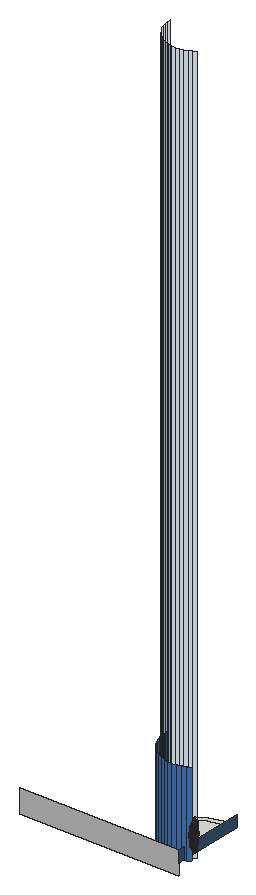
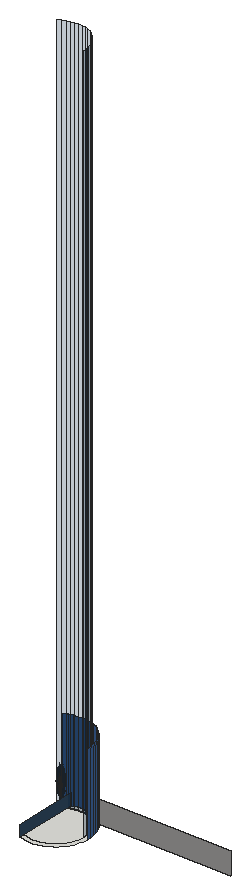
# SketchUp Ruby script. Lengths in inches.
U = 1.inch
M = Sketchup.active_model
def pt(a) = Geom::Point3d.new(a.map { |v| v * U })
def face(e, loops, mat)
  f = e.add_face(loops[0].map { |a| pt(a) })
  loops[1..].each { |l| e.add_face(l.map { |a| pt(a) }).erase! }
  f.material = f.back_material = mat if mat
  f
end
# faces: each face lists its corners as indices into pts; further lists are holes
def faces(e, pts, list, mat = nil) = list.each { |f| face(e, (f[0].is_a?(Array) ? f : [f]).map { |l| l.map { |i| pts[i] } }, mat) }
# xy, xz, yz: faces in a plane at the given z, y or x. An outline is a flat list of corners, or four numbers for a rectangle; further outlines are holes
def ring(l) = l.size == 4 ? [[l[0], l[1]], [l[2], l[1]], [l[2], l[3]], [l[0], l[3]]] : l.each_slice(2).to_a
def flat(e, list, mat, &to3) = list.each { |f| face(e, (f[0].is_a?(Array) ? f : [f]).map { |l| ring(l).map { |u, v| to3.(u, v) } }, mat) }
def xy(e, z, list, mat = nil) = flat(e, list, mat) { |x, y| [x, y, z] }
def xz(e, y, list, mat = nil) = flat(e, list, mat) { |x, z| [x, y, z] }
def yz(e, x, list, mat = nil) = flat(e, list, mat) { |y, z| [x, y, z] }
def lines(e, pts, list) = list.each { |a, b| e.add_line(pt(pts[a]), pt(pts[b])) }
# prism: a flat outline (further loops are holes) pulled along v
def prism(e, loops, v, mat = nil)
  f = face(e, loops, mat); d = Geom::Vector3d.new(v.map { |x| x * U })
  f.pushpull(f.normal.samedirection?(d) ? d.length : -d.length)
end
def box(e, o, s, mat = nil) = prism(e, [[o, [o[0] + s[0], o[1], o[2]], [o[0] + s[0], o[1] + s[1], o[2]], [o[0], o[1] + s[1], o[2]]]], [0, 0, s[2]], mat)
def at(x, y, z, deg = 0) = Geom::Transformation.translation(pt([x, y, z])) * Geom::Transformation.rotation(ORIGIN, Z_AXIS, deg.degrees)
def axes(o, x, y, z) = Geom::Transformation.new([*x, 0, *y, 0, *z, 0, *pt(o).to_a, 1])
def part(name) = M.definitions.add(name)
# library, detail: a bought-in or finely detailed component or shape, given as its bounding box
def library(name, o, s) = part(name).tap { |d| box(d.entities, o, s) }
def detail(e, o, s) = box(e.add_group.entities, o, s)
def put(e, d, t, mat = nil) = e.add_instance(d, t).tap { |i| i.material = mat if mat }
def group(e, t, mat = nil) = e.add_group.tap { |g| g.transformation = t; g.material = mat if mat }.entities
root = M.entities
M.materials.add("Carpet_01_1K").color = [196, 195, 193]
M.materials.add("Carpet_04_1K").color = [56, 85, 112]
M.materials.add("Glass_Basic_1").color = [0, 47, 91]
M.materials["Glass_Basic_1"].alpha = 0.25
M.materials.add("Glass_Mirror_01").color = [71, 118, 185]
M.materials.add("LightPink_Translucent").color = [144, 107, 117]
M.materials["LightPink_Translucent"].alpha = 0.75
c1 = part("blade")
p = [[2.15,0.21,22],[0,0.17,0],[0.09,0.45,0],[2.18,0.31,22],[2.29,0.31,22],[0.38,0.45,0],
  [2.48,0.24,33],[2.49,0.24,33],[2.48,0.22,33]]
faces(c1.entities,p,[[0,1,2,3],[4,5,2,3],[6,3,4,7],[8,0,3,6]])
c2 = part("seeds")
p = [[0.3,-0.1,1.38],[-0.01,-0.03,1.59],[-0.01,-0.03,0.03],[0.14,-0.07,-0.07],[0.29,-0.03,3],[0.15,0.01,3.11]]
faces(c2.entities,p,[[0,1,2,3],[1,0,4,5]],"LightPink_Translucent")
c3 = part("blade with seeds")
put(c3.entities,c1,at(0,0,0))
put(c3.entities,c2,axes([2.4,0.25,30.99],[1.5799,-0.05474,1.17369],[-0.12525,1.92788,0.29478],[-0.07173,-0.02425,1.56792]))
xy(root,-24,[[308.78,9.74,299.76,10.31,290.875,12,282.28,14.79,274.09,18.64,266.46,23.49,259.49,29.25,253.3,35.84,247.99,43.16,243.63,51.08,240.3,59.49,238.06,68.25,236.92,77.22,236.92,86.26,238.06,95.23,240.3,103.99,243.63,112.39,247.99,120.32,253.3,127.63,259.49,134.22,266.46,139.99,274.09,144.83,282.28,148.68,290.875,151.48,299.76,153.17,308.78,153.74,330.57,149.5,330.57,140.33,308.19,144.68,300.89,144.22,293.12,142.74,285.6,140.3,278.4375,136.93,271.76,132.69,265.67,127.65,260.25,121.88,255.6,115.49,251.79,108.55,248.88,101.2,246.91,93.54,245.92,85.69,245.92,77.78,246.91,69.9375,248.88,62.28,251.79,54.92,255.6,47.99,260.25,41.59,265.67,35.83,271.76,30.78,278.4375,26.55,285.6,23.18,293.12,20.73,300.89,19.25,308.78,18.76,316.67,19.25,324.44,20.73,330.57,22.73,330.57,13.26,326.6875,12,317.8,10.31],[308.78,18.76,300.89,19.25,293.12,20.73,285.6,23.18,278.4375,26.55,271.76,30.78,265.67,35.83,260.25,41.59,255.6,47.99,251.79,54.92,248.88,62.28,246.91,69.9375,245.92,77.78,245.92,85.69,246.91,93.54,248.88,101.2,251.79,108.55,255.6,115.49,260.25,121.88,265.67,127.65,271.76,132.69,278.4375,136.93,285.6,140.3,293.12,142.74,300.89,144.22,308.19,144.68,330.57,140.33,330.57,22.73,324.44,20.73,316.67,19.25]])
xz(root,0,[[0,-48,330.57,0]],"Carpet_01_1K")
yz(root,236.92,[[77.22,-24,86.26,150]],"Glass_Mirror_01")
yz(root,245.92,[[77.78,-24,85.69,1482]],"Glass_Basic_1")
yz(root,330.57,[[0,-24,149.5,0]],"Carpet_04_1K")
p = [[308.78,9.74,-24],[308.78,9.74,150],[299.76,10.3,150],[299.76,10.31,-24],[317.8,10.31,-24],[317.8,10.3,150],
  [290.875,12,150],[290.875,12,-24],[326.6875,12,-24],[326.6875,12,150],[282.28,14.79,150],[282.28,14.79,-24],
  [335.29,14.79,-24],[335.29,14.79,150],[330.57,13.26,-24],[274.09,18.64,150],[274.09,18.64,-24],[343.47,18.64,-24],
  [343.47,18.64,150],[266.46,23.49,150],[266.46,23.49,-24],[300.89,19.25,1482],[308.78,18.76,1482],[308.78,18.76,-24],
  [300.89,19.25,-24],[316.67,19.25,1482],[316.67,19.25,-24],[293.12,20.73,1482],[293.12,20.73,-24],[324.44,20.73,1482],
  [324.44,20.73,-24],[285.6,23.18,1482],[285.6,23.18,-24],[331.97,23.18,1482],[331.97,23.18,-24],[330.57,22.73,-24],
  [278.4375,26.55,1482],[278.4375,26.55,-24],[339.12,26.55,1482],[339.12,26.55,-24],[259.49,29.25,150],[259.49,29.25,-24],
  [271.76,30.78,1482],[271.76,30.78,-24],[345.8,30.78,1482],[345.8,30.78,-24],[253.3,35.84,150],[253.3,35.84,-24],
  [265.67,35.83,1482],[265.67,35.83,-24],[247.99,43.16,150],[247.99,43.16,-24],[260.25,41.59,1482],[260.25,41.59,-24],
  [255.6,47.99,1482],[255.6,47.99,-24],[243.63,51.08,150],[243.63,51.08,-24],[251.79,54.92,1482],[251.79,54.92,-24],
  [240.3,59.49,150],[240.3,59.49,-24],[248.88,62.28,1482],[248.88,62.28,-24],[238.06,68.25,150],[238.06,68.25,-24],
  [246.91,69.9375,1482],[246.91,69.9375,-24],[236.92,77.22,150],[236.92,77.22,-24],[245.92,77.78,1482],[245.92,77.78,-24]]
faces(root,p,[[0,1,2,3],[4,5,1,0],[3,2,6,7],[8,9,5,4],[7,6,10,11],[12,13,9,8,14],[11,10,15,16],[17,18,13,12],
  [16,15,19,20],[20,19,40,41],[41,40,46,47],[47,46,50,51],[51,50,56,57],[57,56,60,61],[61,60,64,65],[65,64,68,69]],"Glass_Mirror_01")
faces(root,p,[[21,22,23,24],[22,25,26,23],[27,21,24,28],[25,29,30,26],[31,27,28,32],[29,33,34,35,30],[36,31,32,37],[33,38,39,34],
  [42,36,37,43],[38,44,45,39],[48,42,43,49],[52,48,49,53],[54,52,53,55],[58,54,55,59],[62,58,59,63],[66,62,63,67],
  [70,66,67,71]],"Glass_Basic_1")
put(root,c3,axes([343.04,21.72,-6.07],[0.14639,-0.01056,1.71376],[-0.09712,0.45778,0.13857],[-0.20862,-0.02831,0.73262]))
put(root,c3,axes([343.1,22.52,-6.07],[0.12246,-0.09864,1.71376],[0.1031,0.45582,0.13857],[-0.19225,0.10302,0.73262]))
put(root,c3,axes([342.72,23.3,-7.36],[0.12266,0.03828,1.43002],[0.07906,0.39104,-0.30754],[-0.16661,0.0732,0.61141]))
put(root,c3,axes([343.8,22.05,-6.61],[0.10032,-0.06746,1.77064],[0.0346,0.47103,0.13857],[-0.2173,0.0625,0.63284]))
put(root,c3,axes([342.72,22.37,-5.23],[-0.05763,0.06055,1.74944],[0.0049,0.44239,-0.27667],[-0.13211,0.05753,0.14031]))
put(root,c3,axes([343.47,21.29,-4.97],[-0.35281,-0.01123,-0.71045],[0.0237,-0.47284,0.08574],[-0.14947,-0.0499,1.00501]))
put(root,c3,axes([343.19,21.41,-7.36],[0.06891,0.12984,1.43002],[-0.15879,0.35293,-0.30754],[-0.16304,-0.08436,0.61141]))
put(root,c3,axes([342.91,22.11,-5.42],[-0.29332,-0.1301,-0.35414],[0.08555,-0.37955,0.4572],[-0.11809,0.0348,0.87481]))
put(root,c3,axes([343.3125,20.98,-6.07],[0.1311,0.08035,1.71376],[-0.27131,0.33708,0.13857],[-0.16909,-0.15206,0.73262]))
put(root,c3,axes([342.08,22.8125,-5.24],[0.04504,0.01251,1.77383],[0.13934,0.41205,-0.16761],[-0.0922,0.10815,0.31391]))
put(root,c3,axes([343.11,22.31,-5.27],[-0.09562,0.42421,-0.51099],[-0.32782,-0.1454,-0.3958],[-0.13199,0.0389,0.97773]))
put(root,c3,axes([343.36,21.39,-5.27],[-0.25628,0.30892,-0.51099],[-0.22444,-0.32634,-0.3958],[-0.13021,-0.047,0.97773]))
put(root,c3,axes([342.94,22.28,-8.46],[0.00895,0.0735,1.76342],[-0.18044,0.38382,-0.26939],[-0.12817,-0.01935,0.30037]))
put(root,c3,axes([343,20.52,-5.24],[0.02617,0.04654,1.77383],[-0.12614,0.41836,-0.16761],[-0.12775,0.00303,0.31391]))
put(root,c3,axes([342.46,24.12,-7.18],[0.14709,-0.21136,1.1486],[0.05804,0.3346,0.84392],[-0.1063,0.05991,0.25299]))
put(root,c3,axes([343.29,20.24,-5.23],[-0.07594,-0.00329,1.74944],[-0.24177,0.32918,-0.27667],[-0.129,-0.06726,0.14031]))
put(root,c3,axes([342.98,22.07,-5.22],[0.09971,-0.42522,0.48003],[0.32782,0.1454,0.3958],[-0.12892,0.02555,0.9933]))
put(root,c3,axes([343.09,21.94,-4.91],[0.17758,0.42229,-0.1216],[-0.31518,0.20752,-0.67495],[-0.13282,0.05572,1.02557]))
put(root,c3,axes([343.49,21.07,-4.91],[-0.0189,0.47427,-0.1216],[-0.35781,-0.01296,-0.67495],[-0.13781,-0.03295,1.02557]))
put(root,c3,axes([343.26,21.1,-5.42],[-0.20082,-0.29199,-0.35414],[0.2293,-0.2764,0.4572],[-0.1165,-0.04206,0.87481]))
put(root,c3,axes([342.95,21.95,-5.22],[-0.12963,-0.31798,0.0643],[0.23638,-0.15564,0.50621],[-0.1042,0.03071,0.77189]))
put(root,c3,axes([343.55,22.83,-6.07],[0.08815,-0.14329,1.71376],[0.22258,0.38678,0.13857],[-0.15267,0.17614,0.73262]))
put(root,c3,axes([343.01,23.21,-5.42],[-0.30722,0.06665,-0.35414],[-0.08112,-0.381,0.4572],[-0.08804,0.10234,0.87481]))
put(root,c3,axes([342.85,24.34,-8.46],[0.04734,0.04659,1.76342],[0.08027,0.4317,-0.26939],[-0.10492,0.09206,0.30037]))
put(root,c3,axes([342.78,21.8,-7.18],[0.22533,-0.03337,1.1486],[-0.14293,0.29403,0.84392],[-0.11135,-0.04411,0.25299]))
put(root,c3,axes([343.05,23.125,-5.22],[-0.08753,-0.42921,0.48003],[0.34336,-0.07449,0.3958],[-0.1012,0.10094,0.9933]))
put(root,c3,axes([343.23,20.99,-4.86],[0.29147,-0.34417,0.53763],[0.25138,0.3655,0.4433],[-0.13675,-0.06349,1.11249]))
put(root,c3,axes([342.99,23.04,-5.22],[-0.2423,-0.19613,0.0643],[0.14107,-0.2793,0.50621],[-0.07768,0.0903,0.77189]))
put(root,c3,axes([343.48,23.19,-6.07],[0.06572,-0.16029,1.71376],[0.27569,0.33172,0.13857],[-0.12437,0.20675,0.73262]))
put(root,c3,axes([343.22,22.07,-4.9],[0.29332,0.1301,0.35414],[-0.08555,0.37955,-0.4572],[-0.11809,0.0348,0.87481]))
put(root,c3,axes([343.27,23.25,-5.27],[0.09067,0.42583,-0.51099],[-0.34336,0.07449,-0.3958],[-0.0984,0.11438,0.97773]))
put(root,c3,axes([343.36,20.99,-5.22],[0.01777,-0.35463,0.0643],[0.26836,0.00972,0.50621],[-0.1028,-0.03711,0.77189]))
put(root,c3,axes([342.73,24.02,-5.23],[-0.00877,0.09229,1.74944],[0.24897,0.32105,-0.27667],[-0.06518,0.15182,0.14031]))
put(root,c3,axes([344.125,22.95,-7.89],[-0.36714,-0.07646,-0.62353],[0.07747,-0.47163,-0.16365],[-0.10956,-0.05715,1.37633]))
put(root,c3,axes([344.19,20.375,-4.52],[-0.23555,0.44708,-0.13619],[-0.34112,-0.25757,-0.75594],[-0.11858,-0.12631,1.14864]))
put(root,c3,axes([343.55,21.25,-4.9],[0.20082,0.29199,0.35414],[-0.2293,0.2764,-0.4572],[-0.1165,-0.04206,0.87481]))
put(root,c3,axes([344.09,20.74,-4.97],[-0.30095,-0.22541,-0.71045],[0.21388,-0.395,0.08574],[-0.10904,-0.13459,1.00501]))
put(root,c3,axes([343.95,20.75,-5.27],[-0.34827,0.11086,-0.51099],[-0.06092,-0.41983,-0.3958],[-0.09354,-0.12031,0.97773]))
put(root,c3,axes([343.64,23.84,-7.93],[-0.33032,-0.23318,-0.49651],[0.19744,-0.41812,0],[-0.07523,-0.05311,1.57504]))
put(root,c3,axes([343.5,20.37,-8.46],[-0.03419,0.06144,1.76342],[-0.3455,0.13246,-0.26939],[-0.08346,-0.12049,0.30037]))
put(root,c3,axes([343.11,22.95,-4.91],[0.32648,0.25715,-0.1216],[-0.18809,0.3724,-0.67495],[-0.09224,0.12945,1.02557]))
put(root,c3,axes([343.84,24.12,-7.58],[-0.22066,0.46731,0],[-0.36918,-0.26061,-0.51607],[-0.08408,-0.05936,1.63711]))
put(root,c3,axes([342.57,24.0625,-4.3],[0.31145,0.12449,-0.06488],[-0.0958,0.38314,-0.29416],[-0.05094,0.05817,0.97024]))
put(root,c3,axes([343.27,22.98,-4.9],[0.30722,-0.06665,0.35414],[0.08112,0.381,-0.4572],[-0.08804,0.10234,0.87481]))
put(root,c3,axes([343.44,24.8,-7.36],[0.11138,-0.07357,1.43002],[0.27499,0.22183,-0.30754],[-0.08185,0.19194,0.61141]))
put(root,c3,axes([343.28,20.6,-7.82],[-0.10181,0.3808,-0.03893],[-0.31336,-0.11714,-0.17649],[-0.04758,-0.06228,0.58215]))
put(root,c3,axes([344.1,19.31,-5.24],[-0.00658,0.0559,1.77383],[-0.32474,0.20287,-0.16761],[-0.09556,-0.1037,0.31391]))
put(root,c3,axes([343.75,20.12,-7.36],[-0.02137,0.15256,1.43002],[-0.31245,0.12771,-0.30754],[-0.07303,-0.19719,0.61141]))
put(root,c3,axes([343.85,20.52,-6.07],[0.08068,0.14973,1.71376],[-0.3728,0.12606,0.13857],[-0.08426,-0.23506,0.73262]))
put(root,c3,axes([344.54,23.02,-7.28],[-0.35635,0.30962,-0.29095],[-0.23697,-0.43749,-0.50002],[-0.08792,-0.04443,1.59708]))
put(root,c3,axes([343.56,23.99,-5.22],[-0.25132,-0.3182,0.48003],[0.2669,-0.27442,0.3958],[-0.04636,0.14929,0.9933]))
put(root,c3,axes([343.98,20.4375,-5.42],[-0.05451,-0.37564,-0.35414],[0.31161,-0.09919,0.4572],[-0.0837,-0.10765,0.87481]))
put(root,c3,axes([343.11,22.34,-7.58],[-0.44133,0,0],[0,-0.52122,-0.51607],[0,-0.11871,1.63711]))
put(root,c3,axes([343.73,23.66,-7.92],[-0.08291,-0.40636,-0.30978],[0.32928,-0.11539,0.30978],[-0.06638,-0.04686,1.38974]))
put(root,c3,axes([343.46,23.96,-5.22],[-0.29004,-0.02173,0.0643],[0.00795,-0.32812,0.50621],[-0.03035,0.12569,0.77189]))
put(root,c3,axes([343.56,24.09,-5.42],[-0.23881,0.24554,-0.35414],[-0.22606,-0.28036,0.4572],[-0.0344,0.14245,0.87481]))
put(root,c3,axes([344.78,23.35,-7.89],[-0.23773,0.35053,-0.62353],[-0.29532,-0.31785,-0.16365],[-0.09526,0.08744,1.37633]))
put(root,c3,axes([344.17,20.74,-4.9],[0.05451,0.37564,0.35414],[-0.31161,0.09919,-0.4572],[-0.0837,-0.10765,0.87481]))
put(root,c3,axes([342.7,24.96,-5.24],[0.04004,-0.02816,1.77383],[0.33095,0.18728,-0.16761],[-0.00778,0.15594,0.31391]))
put(root,c3,axes([343.46,22.2,-7.62],[-0.32829,0.39208,0.30756],[-0.32849,-0.38796,-0.36492],[-0.01146,-0.11134,1.64885]))
put(root,c3,axes([344.81,23.29,-6.625],[0.305,0.18805,1.51261],[-0.29879,0.40513,0.59816],[-0.13384,-0.24012,1.26806]))
put(root,c3,axes([343.64,19.875,-7.18],[0.18411,0.16231,1.1486],[-0.26813,0.09757,0.84392],[-0.05737,-0.12474,0.25299]))
put(root,c3,axes([344.94,23.16,-7.48],[-0.34464,-0.37536,-0.25192],[0.29,-0.42149,0.5513],[-0.0928,0.04391,1.68216]))
put(root,c3,axes([344.31,22.8,-7.74],[-0.21202,-0.39143,-0.44739],[0.32115,-0.27564,0.21531],[-0.06861,-0.04843,1.43643]))
put(root,c3,axes([343.71,23.83,-4.61],[-0.00918,0.43138,-0.7886],[-0.38672,-0.02897,0.09517],[-0.04081,0.18275,1.11556]))
put(root,c3,axes([343.71,25.04,-7.18],[-0.00913,-0.2773,1.1486],[0.22824,0.19778,0.84392],[-0.04489,0.13217,0.25299]))
put(root,c3,axes([344.03,20.3,-4.86],[0.39316,-0.11987,0.53763],[0.06823,0.47021,0.4433],[-0.09247,-0.13858,1.11249]))
put(root,c3,axes([344.77,23.08,-7.74],[-0.38326,0.02879,-0.44739],[-0.03466,-0.47788,0.21531],[-0.06861,0.04843,1.43643]))
put(root,c3,axes([344.12,20.4,-5.22],[0.16041,-0.29625,0.0643],[0.22843,0.17248,0.50621],[-0.07385,-0.09498,0.77189]))
put(root,c3,axes([344.03,23.875,-7.47],[0.33032,0.23318,0.49651],[-0.19744,0.41812,0],[-0.07523,-0.05311,1.57504]))
put(root,c3,axes([343.59,24.4375,-6.59],[0.00775,-0.24075,1.54345],[0.34877,0.12716,0.21329],[-0.03022,0.25658,0.72882]))
put(root,c3,axes([344.35,23.02,-7.51],[0.09355,-0.55261,-0.23429],[0.44354,0.09633,0.51271],[-0.0775,-0.07631,1.5644]))
put(root,c3,axes([344.51,23.15,-7.33],[-0.06809,0.4162,0.1448],[-0.33266,-0.07225,-0.41347],[-0.06054,-0.04274,1.26744]))
put(root,c3,axes([344.47,19.52,-5.23],[-0.05398,-0.06539,1.74944],[-0.36026,0.04145,-0.27667],[-0.0575,-0.15639,0.14031]))
put(root,c3,axes([345.17,24.31,-7.93],[-0.33032,0.23318,-0.49651],[-0.19744,-0.41812,0],[-0.07523,0.05311,1.57504]))
put(root,c3,axes([343.21,21.99,-7.93],[0,-0.46636,-0.49651],[0.39487,0,0],[0,-0.10622,1.57504]))
put(root,c3,axes([343.38,22.42,-7.47],[0,0.46636,0.49651],[-0.39487,0,0],[0,-0.10622,1.57504]))
put(root,c3,axes([345.19,24.19,-7.76],[-0.21791,-0.46895,-0.05142],[0.36918,-0.26061,0.51607],[-0.09097,0.04465,1.6363]))
put(root,c3,axes([343.79,23.97,-4.94],[0.25266,0.31335,-0.5672],[-0.2669,0.27442,-0.43934],[-0.03844,0.15921,1.08528]))
put(root,c3,axes([345.09,24.125,-7.92],[-0.32928,-0.11539,-0.30978],[0.08291,-0.40636,0.30978],[-0.06638,0.04686,1.38974]))
put(root,c3,axes([343.68,23.74,-4.9],[0.23881,-0.24554,0.35414],[0.22606,0.28036,-0.4572],[-0.0344,0.14245,0.87481]))
put(root,c3,axes([344.25,22.53,-7.28],[-0.39748,-0.22252,-0.29095],[0.19139,-0.46966,-0.50002],[-0.01249,-0.11531,1.59708]))
put(root,c3,axes([345.28,22.39,-7.11],[-0.00964,-0.43909,1.41272],[0.43635,0.11382,0.59816],[-0.1032,0.24027,1.3335]))
put(root,c3,axes([343.53,23.81,-4.55],[0.3879,0.02311,-0.13498],[-0.0106,0.43749,-0.74919],[-0.02694,0.1685,1.13838]))
put(root,c3,axes([343.52,24.44,-7.125],[0.32063,-0.08258,0.06507],[0.07371,0.33271,-0.86304],[-0.02033,0.16842,0.7736]))
put(root,c3,axes([345.04,22.95,-7.28],[0.04113,0.53214,-0.29095],[-0.42835,0.03218,-0.50002],[-0.07543,0.07088,1.59708]))
put(root,c3,axes([344.07,22.05,-7.85],[-0.14494,-0.47823,-0.69835],[0.41752,-0.17223,-0.18329],[-0.01602,-0.16194,1.54149]))
put(root,c3,axes([345.02,20.53,-4.91],[-0.34538,0.21713,-0.1216],[-0.16972,-0.38536,-0.67495],[-0.04557,-0.16239,1.02557]))
put(root,c3,axes([344.72,20.55,-5.27],[-0.34695,-0.11691,-0.51099],[0.11892,-0.40083,-0.3958],[-0.03181,-0.16138,0.97773]))
put(root,c3,axes([344.08,23.52,-6.07],[-0.00864,-0.17899,1.71376],[0.37441,0.11874,0.13857],[-0.02316,0.25508,0.73262]))
put(root,c3,axes([343.38,22,-7.92],[0.24637,-0.29097,-0.30978],[0.24637,0.29097,0.30978],[0,-0.09372,1.38974]))
put(root,c3,axes([344.5,20.12,-7.82],[-0.2439,0.26754,-0.03893],[-0.22348,-0.29302,-0.17649],[-0.01573,-0.08303,0.58215]))
put(root,c3,axes([344.4,22.75,-7.59],[0.44609,0.09826,0.45755],[-0.09078,0.55493,0.17955],[-0.06519,-0.05359,1.58856]))
put(root,c3,axes([344.28,22.65,-7.23],[-0.17124,0.42022,0.44739],[-0.35581,-0.20224,-0.21531],[0,-0.09687,1.43643]))
put(root,c3,axes([344.85,20.63,-4.97],[-0.16845,-0.3792,-0.71045],[0.34676,-0.21133,0.08574],[-0.03939,-0.18322,1.00501]))
put(root,c3,axes([344.16,23.64,-7.47],[0.37926,-0.12378,0.17642],[0.09365,0.46065,0.35086],[-0.03382,-0.06712,1.60407]))
put(root,c3,axes([344.65,23.71,-7.75],[-0.35581,-0.20937,0],[0.17124,-0.43505,0],[0,0,1.62707]))
put(root,c3,axes([344.91,20.68,-4.9],[-0.1064,0.35863,0.35414],[-0.31043,-0.1046,-0.4572],[-0.02846,-0.14439,0.87481]))
put(root,c3,axes([345.47,24.24,-7.58],[0.22066,0.46731,0],[-0.36918,0.26061,-0.51607],[-0.08408,0.05936,1.63711]))
put(root,c3,axes([344.35,24.4375,-4.89],[-0.34777,-0.12192,0.53283],[0.11892,-0.40083,0.43934],[0.0209,0.15763,1.10256]))
put(root,c3,axes([344.25,24.47,-5.22],[-0.26007,0.1585,0.0643],[-0.12729,-0.28902,0.50621],[0.02512,0.1274,0.77189]))
put(root,c3,axes([345.29,23.67,-7.47],[0.10196,-0.46348,0.17642],[0.3731,0.13116,0.35086],[-0.06445,0.00226,1.60407]))
put(root,c3,axes([345.11,23.05,-7.33],[0.26075,0.2802,0.1448],[-0.2175,0.31612,-0.41347],[-0.06054,0.04274,1.26744]))
put(root,c3,axes([345.02,22.71,-7.65],[-0.32829,-0.4014,-0.06131],[0.32849,-0.40164,0],[-0.01146,-0.01402,1.75571]))
put(root,c3,axes([345.11,22.85,-7.23],[0.38326,-0.02879,0.44739],[0.03466,0.47788,-0.21531],[-0.06861,0.04843,1.43643]))
put(root,c3,axes([345.2,23.94,-7.62],[0.44186,0.15158,0.30756],[-0.11054,0.54181,-0.36492],[-0.07313,0.06781,1.64885]))
put(root,c3,axes([344.56,19.79,-8.46],[-0.0592,0.0168,1.76342],[-0.32738,-0.18913,-0.26939],[0.00549,-0.15776,0.30037]))
put(root,c3,axes([345.39,23.91,-7.47],[0.33032,-0.23318,0.49651],[0.19744,0.41812,0],[-0.07523,0.05311,1.57504]))
put(root,c3,axes([344.88,20.31,-5.42],[0.1064,-0.35863,-0.35414],[0.31043,0.1046,0.4572],[-0.02846,-0.14439,0.87481]))
put(root,c3,axes([344.36,22.24,-7.59],[0.15345,0.52148,0.45755],[-0.43845,0.18134,0.17955],[0.00536,-0.09582,1.58856]))
put(root,c3,axes([344.29,22.18,-7.74],[0.17124,-0.42022,-0.44739],[0.35581,0.20224,0.21531],[0,-0.09687,1.43643]))
put(root,c3,axes([344.73,23.53,-7.75],[-0.11516,-0.40207,0],[0.32884,-0.1408,0],[0,0,1.54371]))
put(root,c3,axes([344.31,24.38,-8.46],[0.05712,-0.02538,1.76342],[0.34359,0.13968,-0.26939],[0.01005,0.15742,0.30037]))
put(root,c3,axes([344.38,24.52,-5.42],[-0.1064,0.35863,-0.35414],[-0.31043,-0.1046,0.4572],[0.02846,0.14439,0.87481]))
put(root,c3,axes([345.19,22.74,-7.74],[-0.17124,0.42022,-0.44739],[-0.35581,-0.20224,0.21531],[0,0.09687,1.43643]))
put(root,c3,axes([345.01,20.36,-5.22],[0.26007,-0.1585,0.0643],[0.12729,0.28902,0.50621],[-0.02512,-0.1274,0.77189]))
put(root,c3,axes([344.16,25.16,-5.23],[0.04474,0.0751,1.74944],[0.36104,0.0295,-0.27667],[0.03631,0.16562,0.14031]))
put(root,c3,axes([345.87,22.48,-7.47],[-0.2773,-0.3397,0.17642],[0.27945,-0.32949,0.35086],[-0.03063,0.06937,1.60407]))
put(root,c3,axes([344.91,22.29,-7.74],[0,-0.53961,0],[0.44133,0,0],[0,0,1.79456]))
put(root,c3,axes([344.92,20.39,-5.22],[0.34777,0.12192,0.48003],[-0.11892,0.40083,0.3958],[-0.0209,-0.15763,0.9933]))
put(root,c3,axes([344.5,22.39,-7.52],[0.39767,0.22603,0.24065],[-0.19139,0.46966,0.50002],[0,-0.10827,1.60543]))
put(root,c3,axes([345.13,22.5,-7.66],[0,0.53934,-0.05637],[-0.44133,0,0],[0,0.01695,1.79368]))
put(root,c3,axes([344.37,22.07,-7.23],[-0.38326,0.02879,0.44739],[-0.03466,-0.47788,-0.21531],[0.06861,-0.04843,1.43643]))
put(root,c3,axes([344.35,24.14,-4.9],[0.1064,-0.35863,0.35414],[0.31043,0.1046,-0.4572],[0.02846,0.14439,0.87481]))
put(root,c3,axes([344.19,21.25,-7.47],[-0.10196,0.46348,0.17642],[-0.3731,-0.13116,0.35086],[0.06445,-0.00226,1.60407]))
put(root,c3,axes([344.92,23.55,-7.66],[0.15345,0.53576,-0.06012],[-0.43845,0.18773,0],[0.00536,0.01871,1.72173]))
put(root,c3,axes([344.01,20.68,-7.58],[-0.22066,-0.46731,0],[0.36918,-0.26061,-0.51607],[0.08408,-0.05936,1.63711]))
put(root,c3,axes([344.42,24.2,-4.97],[0.16845,0.3792,-0.71045],[-0.34676,0.21133,0.08574],[0.03939,0.18322,1.00501]))
put(root,c3,axes([346.1875,22.84,-7.75],[-0.44111,-0.00373,-0.04976],[0,-0.52122,0.49943],[-0.01386,0.11865,1.58352]))
put(root,c3,axes([345.32,21.28,-7.47],[-0.37926,0.12378,0.17642],[-0.09365,-0.46065,0.35086],[0.03382,0.06712,1.60407]))
put(root,c3,axes([344.93,19.55,-7.18],[0.04528,0.27194,1.1486],[-0.25117,-0.15062,0.84392],[0.02703,-0.13924,0.25299]))
put(root,c3,axes([344.77,25.42,-4.3],[0.2439,-0.26754,-0.06488],[0.22348,0.29302,-0.29416],[0.01573,0.08303,0.97024]))
put(root,c3,axes([344.7,21.95,-7.59],[-0.29264,0.42323,0.45755],[-0.34767,-0.3736,0.17955],[0.07055,-0.04224,1.58856]))
put(root,c3,axes([345.2,22.62,-7.73],[0.24637,0.30123,0],[-0.24637,0.30123,0],[0,0,1.69266]))
put(root,c3,axes([345.2,22.26,-7.23],[0.17124,-0.42022,0.44739],[0.35581,0.20224,-0.21531],[0,0.09687,1.43643]))
put(root,c3,axes([345.05,23.72,-7.75],[0.35581,0.20937,0],[-0.17124,0.43505,0],[0,0,1.74954]))
put(root,c3,axes([344.54,24.28,-5.27],[0.34695,0.11691,-0.51099],[-0.11892,0.40083,-0.3958],[0.03181,0.16138,0.97773]))
put(root,c3,axes([344.25,24.3,-4.91],[0.34538,-0.21713,-0.1216],[0.16972,0.38536,-0.67495],[0.04557,0.16239,1.02557]))
put(root,c3,axes([345.08,22.16,-7.57],[-0.44609,-0.09826,0.49198],[0.09078,-0.55493,0.19306],[0.06519,0.05359,1.70813]))
put(root,c3,axes([346.01,19.99,-5.24],[-0.03584,0.03562,1.77383],[-0.35118,-0.12018,-0.16761],[-0.01271,-0.15545,0.31391]))
put(root,c3,axes([345.73,21.02,-4.91],[-0.3879,-0.02311,-0.1216],[0.0106,-0.43749,-0.67495],[0.02694,-0.1685,1.02557]))
put(root,c3,axes([346.1,22.92,-7.92],[-0.24637,0.29097,-0.30978],[-0.24637,-0.29097,0.30978],[0,0.09372,1.38974]))
put(root,c3,axes([345.39,22.87,-7.85],[0.12941,0.42699,-0.69212],[-0.37279,0.15378,-0.18165],[0.0143,0.14459,1.52773]))
put(root,c3,axes([345.21,22.41,-7.74],[0.39487,0,0],[0,0.48281,0],[0,0,1.78407]))
put(root,c3,axes([345.58,21.09,-4.9],[-0.23881,0.24554,0.35414],[-0.22606,-0.28036,-0.4572],[0.0344,-0.14245,0.87481]))
put(root,c3,axes([344.83,21.875,-7.23],[-0.21202,-0.39143,0.44739],[0.32115,-0.27564,-0.21531],[0.06861,0.04843,1.43643]))
put(root,c3,axes([344.44,21.97,-7.28],[-0.04113,-0.53214,-0.29095],[0.42835,-0.03218,-0.50002],[0.07543,-0.07088,1.59708]))
put(root,c3,axes([345.35,22.36,-7.33],[0.32884,-0.136,0.1448],[0.11516,0.38837,-0.41347],[0,0.08547,1.26744]))
put(root,c3,axes([345.47,20.86,-5.27],[-0.25266,-0.31335,-0.51099],[0.2669,-0.27442,-0.3958],[0.03844,-0.15921,0.97773]))
put(root,c3,axes([345.23,22.39,-7.28],[0.39748,0.22252,-0.29095],[-0.19139,0.46966,-0.50002],[0.01249,0.11531,1.59708]))
put(root,c3,axes([344.39,20.79,-7.92],[0.32928,0.11539,-0.30978],[-0.08291,0.40636,0.30978],[0.06638,-0.04686,1.38974]))
put(root,c3,axes([345.3,20.3,-7.36],[-0.10032,0.0944,1.43002],[-0.30046,-0.16522,-0.30754],[0.05569,-0.20547,0.61141]))
put(root,c3,axes([346.1,22.5,-7.47],[0,-0.46636,0.49651],[0.39487,0,0],[0,0.10622,1.57504]))
put(root,c3,axes([346.27,22.93,-7.93],[0,0.46636,-0.49651],[-0.39487,0,0],[0,0.10622,1.57504]))
put(root,c3,axes([345.21,24.34,-5.22],[-0.35104,0.10702,0.48003],[-0.06092,-0.41983,0.3958],[0.08256,0.12373,0.9933]))
put(root,c3,axes([344.3125,20.61,-7.93],[0.33032,-0.23318,-0.49651],[0.19744,0.41812,0],[0.07523,-0.05311,1.57504]))
put(root,c3,axes([345.14,24.43,-5.22],[-0.16041,0.29625,0.0643],[-0.22843,-0.17248,0.50621],[0.07385,0.09498,0.77189]))
put(root,c3,axes([344.74,23.45,-6.07],[-0.08068,-0.14973,1.71376],[0.3728,-0.12606,0.13857],[0.08426,0.23506,0.73262]))
put(root,c3,axes([344.97,21.77,-7.33],[0.06809,-0.4162,0.1448],[0.33266,0.07225,-0.41347],[0.06054,0.04274,1.26744]))
put(root,c3,axes([345.45,21.04,-7.47],[-0.33032,-0.23318,0.49651],[0.19744,-0.41812,0],[0.07523,0.05311,1.57504]))
put(root,c3,axes([345.55,21,-4.97],[0.00918,-0.43138,-0.71045],[0.38672,0.02897,0.08574],[0.04081,-0.18275,1.00501]))
put(root,c3,axes([345.16,23.48,-7.76],[0.37054,-0.15823,-0.19198],[0.1302,0.45581,0.00008],[0.0409,-0.01749,1.73897]))
put(root,c3,axes([345.1,24.09,-4.9],[-0.05451,-0.37564,0.35414],[0.31161,-0.09919,-0.4572],[0.0837,0.10765,0.87481]))
put(root,c3,axes([345.16,22.12,-7.74],[0.21202,0.39143,-0.44739],[-0.32115,0.27564,0.21531],[0.06861,0.04843,1.43643]))
put(root,c3,axes([345.3,21.92,-5.48],[-0.30498,-0.24231,1.38283],[0.32203,-0.37727,0.59665],[0.0984,0.22736,1.33663]))
put(root,c3,axes([345.71,20.74,-5.42],[0.23881,-0.24554,-0.35414],[0.22606,0.28036,0.4572],[0.0344,-0.14245,0.87481]))
put(root,c3,axes([344.79,24.61,-5.24],[0.00104,-0.05646,1.77383],[0.30246,-0.2491,-0.16761],[0.10506,0.08891,0.31391]))
put(root,c3,axes([345.8,20.87,-5.22],[0.29004,0.02173,0.0643],[-0.00795,0.32812,0.50621],[0.03035,-0.12569,0.77189]))
put(root,c3,axes([345.76,23.9,-7.18],[-0.19872,-0.13409,1.1486],[0.2566,-0.13625,0.84392],[0.06921,0.11541,0.25299]))
put(root,c3,axes([345.06,23.75,-7.36],[0.00623,-0.15459,1.43002],[0.29764,-0.17268,-0.30754],[0.09188,0.18503,0.61141]))
